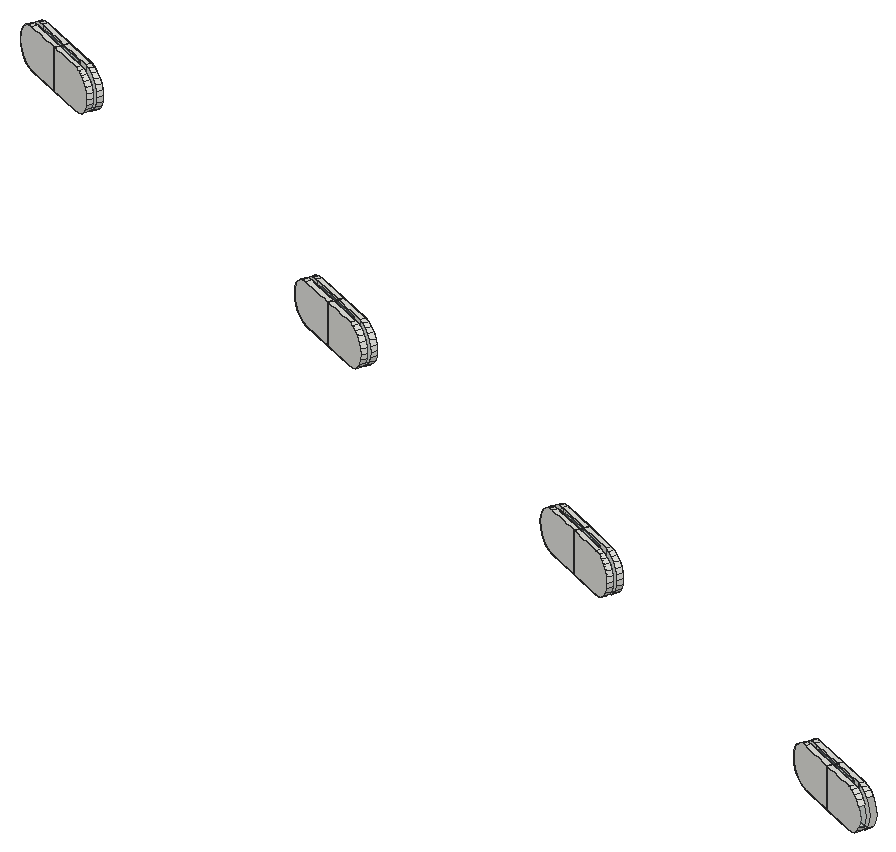
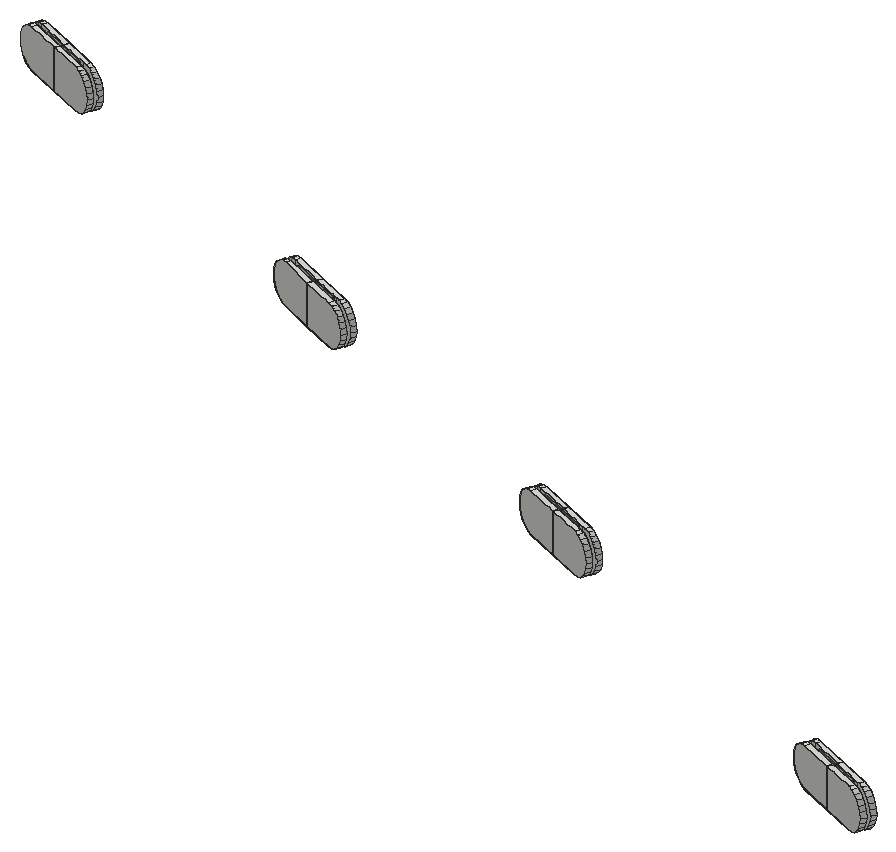
# SketchUp Ruby script. Lengths in inches.
U = 1.inch
M = Sketchup.active_model
def pt(a) = Geom::Point3d.new(a.map { |v| v * U })
def face(e, loops, mat)
  f = e.add_face(loops[0].map { |a| pt(a) })
  loops[1..].each { |l| e.add_face(l.map { |a| pt(a) }).erase! }
  f.material = f.back_material = mat if mat
  f
end
# faces: each face lists its corners as indices into pts; further lists are holes
def faces(e, pts, list, mat = nil) = list.each { |f| face(e, (f[0].is_a?(Array) ? f : [f]).map { |l| l.map { |i| pts[i] } }, mat) }
# xy, xz, yz: faces in a plane at the given z, y or x. An outline is a flat list of corners, or four numbers for a rectangle; further outlines are holes
def ring(l) = l.size == 4 ? [[l[0], l[1]], [l[2], l[1]], [l[2], l[3]], [l[0], l[3]]] : l.each_slice(2).to_a
def flat(e, list, mat, &to3) = list.each { |f| face(e, (f[0].is_a?(Array) ? f : [f]).map { |l| ring(l).map { |u, v| to3.(u, v) } }, mat) }
def xy(e, z, list, mat = nil) = flat(e, list, mat) { |x, y| [x, y, z] }
def xz(e, y, list, mat = nil) = flat(e, list, mat) { |x, z| [x, y, z] }
def yz(e, x, list, mat = nil) = flat(e, list, mat) { |y, z| [x, y, z] }
def lines(e, pts, list) = list.each { |a, b| e.add_line(pt(pts[a]), pt(pts[b])) }
# prism: a flat outline (further loops are holes) pulled along v
def prism(e, loops, v, mat = nil)
  f = face(e, loops, mat); d = Geom::Vector3d.new(v.map { |x| x * U })
  f.pushpull(f.normal.samedirection?(d) ? d.length : -d.length)
end
def box(e, o, s, mat = nil) = prism(e, [[o, [o[0] + s[0], o[1], o[2]], [o[0] + s[0], o[1] + s[1], o[2]], [o[0], o[1] + s[1], o[2]]]], [0, 0, s[2]], mat)
def at(x, y, z, deg = 0) = Geom::Transformation.translation(pt([x, y, z])) * Geom::Transformation.rotation(ORIGIN, Z_AXIS, deg.degrees)
def axes(o, x, y, z) = Geom::Transformation.new([*x, 0, *y, 0, *z, 0, *pt(o).to_a, 1])
def part(name) = M.definitions.add(name)
# library, detail: a bought-in or finely detailed component or shape, given as its bounding box
def library(name, o, s) = part(name).tap { |d| box(d.entities, o, s) }
def detail(e, o, s) = box(e.add_group.entities, o, s)
def put(e, d, t, mat = nil) = e.add_instance(d, t).tap { |i| i.material = mat if mat }
def group(e, t, mat = nil) = e.add_group.tap { |g| g.transformation = t; g.material = mat if mat }.entities
root = M.entities
M.materials.add("Glass_Safety_01").color = [204, 235, 244]
M.materials["Glass_Safety_01"].alpha = 0.1
xy(root,333,[[788.71,557.36,786.9,558.15,787.01,558.4,788.82,557.62],[788.9,557.8,787.09,558.58,787.2,558.84,789.01,558.05],[786.9,558.15,785.1,558.9375,785.21,559.1875,785.36,559.12,787.01,558.4],[787.09,558.58,785.44,559.3,785.29,559.37,785.4,559.62,787.2,558.84],[767.73,566.5,765.93,567.29,766.04,567.54,767.84,566.75],
  [767.92,566.93,766.12,567.72,766.23,567.97,768.03,567.19],[765.93,567.29,764.12,568.07,764.23,568.32,764.39,568.25,766.04,567.54],[766.12,567.72,764.47,568.43,764.3125,568.5,764.42,568.76,766.23,567.97],[747.39,575.36,745.58,576.15,745.69,576.4,747.5,575.61],[747.57,575.79,745.77,576.58,745.88,576.83,747.68,576.05],
  [745.58,576.15,743.78,576.93,743.89,577.19,744.03,577.12,745.69,576.4],[745.77,576.58,744.11,577.3,743.96,577.37,744.07,577.62,745.88,576.83],[724.68,585.25,722.875,586.04,722.99,586.29,724.79,585.5],[724.87,585.68,723.0625,586.47,723.17,586.72,724.98,585.94],[722.875,586.04,721.07,586.82,721.18,587.07,721.33,587.01,722.99,586.29],
  [723.0625,586.47,721.4,587.19,721.26,587.25,721.37,587.51,723.17,586.72]])
xy(root,333.08,[[788.46,557.77,787.01,558.4,787.09,558.58,788.54,557.95],[787.01,558.4,785.57,559.03,785.65,559.21,787.09,558.58],[767.48,566.91,766.04,567.54,766.12,567.72,767.56,567.09],[766.04,567.54,764.59,568.17,764.67,568.35,766.12,567.72],[747.13,575.77,745.69,576.4,745.77,576.58,747.21,575.95],
  [745.69,576.4,744.25,577.03,744.33,577.21,745.77,576.58],[724.43,585.66,722.99,586.29,723.0625,586.47,724.51,585.84],[722.99,586.29,721.54,586.92,721.62,587.1,723.0625,586.47]],"Glass_Safety_01")
xy(root,335.05,[[788.46,557.77,788.54,557.95,787.09,558.58,787.01,558.4],[787.01,558.4,787.09,558.58,785.65,559.21,785.57,559.03],[767.48,566.91,767.56,567.09,766.12,567.72,766.04,567.54],[766.04,567.54,766.12,567.72,764.67,568.35,764.59,568.17],[747.13,575.77,747.21,575.95,745.77,576.58,745.69,576.4],
  [745.69,576.4,745.77,576.58,744.33,577.21,744.25,577.03],[724.43,585.66,724.51,585.84,723.0625,586.47,722.99,586.29],[722.99,586.29,723.0625,586.47,721.62,587.1,721.54,586.92]],"Glass_Safety_01")
xy(root,335.125,[[788.71,557.36,788.82,557.62,787.01,558.4,786.9,558.15],[788.9,557.8,789.01,558.05,787.2,558.84,787.09,558.58],[786.9,558.15,787.01,558.4,785.36,559.12,785.21,559.1875,785.1,558.9375],[787.09,558.58,787.2,558.84,785.4,559.62,785.29,559.37,785.44,559.3],[767.73,566.5,767.84,566.75,766.04,567.54,765.93,567.29],
  [767.92,566.93,768.03,567.19,766.23,567.97,766.12,567.72],[765.93,567.29,766.04,567.54,764.39,568.25,764.23,568.32,764.12,568.07],[766.12,567.72,766.23,567.97,764.42,568.76,764.3125,568.5,764.47,568.43],[747.39,575.36,747.5,575.61,745.69,576.4,745.58,576.15],[747.57,575.79,747.68,576.05,745.88,576.83,745.77,576.58],
  [745.58,576.15,745.69,576.4,744.03,577.12,743.89,577.19,743.78,576.93],[745.77,576.58,745.88,576.83,744.07,577.62,743.96,577.37,744.11,577.3],[724.68,585.25,724.79,585.5,722.99,586.29,722.875,586.04],[724.87,585.68,724.98,585.94,723.17,586.72,723.0625,586.47],[722.875,586.04,722.99,586.29,721.33,587.01,721.18,587.07,721.07,586.82],
  [723.0625,586.47,723.17,586.72,721.37,587.51,721.26,587.25,721.4,587.19]])
p = [[788.71,557.36,335.125],[786.9,558.15,335.125],[786.9,558.15,333],[788.71,557.36,333],[788.96,557.25,333.04],[789.2,557.15,333.14],
  [789.4,557.0625,333.3125],[789.55,557,333.53],[789.65,556.95,333.79],[789.68,556.9375,334.0625],[789.65,556.95,334.34],[789.55,557,334.59],
  [789.4,557.0625,334.8125],[789.2,557.15,334.98],[788.96,557.25,335.09],[788.82,557.62,335.125],[788.82,557.62,333],[789.07,557.51,333.04],
  [789.31,557.4,333.14],[789.51,557.32,333.3125],[789.66,557.25,333.53],[789.76,557.21,333.79],[789.79,557.19,334.0625],[789.76,557.21,334.34],
  [789.66,557.25,334.59],[789.51,557.32,334.8125],[789.31,557.4,334.98],[789.07,557.51,335.09],[788.9,557.8,333],[788.9,557.8,335.125],
  [789.15,557.6875,335.09],[789.38,557.58,334.98],[789.59,557.5,334.8125],[789.74,557.43,334.59],[789.84,557.39,334.34],[789.87,557.37,334.0625],
  [789.84,557.39,333.79],[789.74,557.43,333.53],[789.59,557.5,333.3125],[789.38,557.58,333.14],[789.15,557.6875,333.04],[787.01,558.4,335.125],
  [787.01,558.4,333],[787.01,558.4,333.08],[788.46,557.77,333.08],[788.46,557.77,335.05],[787.01,558.4,335.05],[787.2,558.84,335.125],
  [789.01,558.05,335.125],[789.26,557.94,335.09],[789.49,557.84,334.98],[789.7,557.75,334.8125],[789.85,557.68,334.59],[789.95,557.64,334.34],
  [789.98,557.625,334.0625],[789.95,557.64,333.79],[789.85,557.68,333.53],[789.7,557.75,333.3125],[789.49,557.84,333.14],[789.26,557.94,333.04],
  [789.01,558.05,333],[787.2,558.84,333],[787.09,558.58,333],[787.09,558.58,335.125],[787.09,558.58,335.05],[788.54,557.95,335.05],
  [788.54,557.95,333.08],[787.09,558.58,333.08],[785.1,558.9375,335.125],[784.85,559.05,335.09],[784.61,559.15,334.98],[784.41,559.24,334.8125],
  [784.25,559.3,334.59],[784.16,559.35,334.34],[784.125,559.36,334.0625],[784.16,559.35,333.79],[784.25,559.3,333.53],[784.41,559.24,333.3125],
  [784.61,559.15,333.14],[784.85,559.05,333.04],[785.1,558.9375,333],[785.36,559.12,333],[785.36,559.12,335.125],[785.57,559.03,335.05],
  [785.57,559.03,333.08],[785.44,559.3,335.125],[785.44,559.3,333],[785.65,559.21,333.08],[785.65,559.21,335.05],[785.4,559.62,335.125],
  [785.4,559.62,333],[785.14,559.73,333.04],[784.91,559.83,333.14],[784.71,559.92,333.3125],[784.55,559.99,333.53],[784.46,560.03,333.79],
  [784.42,560.05,334.0625],[784.46,560.03,334.34],[784.55,559.99,334.59],[784.71,559.92,334.8125],[784.91,559.83,334.98],[785.14,559.73,335.09],
  [784.96,559.3,333.04],[785.21,559.1875,333],[784.72,559.4,333.14],[785.21,559.1875,335.125],[784.52,559.49,333.3125],[784.36,559.56,333.53],
  [784.27,559.6,333.79],[784.23,559.61,334.0625],[784.27,559.6,334.34],[784.36,559.56,334.59],[784.52,559.49,334.8125],[784.72,559.4,334.98],
  [784.96,559.3,335.09],[785.29,559.37,333],[785.29,559.37,335.125],[785.03,559.48,335.09],[784.8,559.58,334.98],[784.6,559.67,334.8125],
  [784.44,559.74,334.59],[784.35,559.78,334.34],[784.3125,559.79,334.0625],[784.35,559.78,333.79],[784.44,559.74,333.53],[784.6,559.67,333.3125],
  [784.8,559.58,333.14],[785.03,559.48,333.04],[767.73,566.5,335.125],[765.93,567.29,335.125],[765.93,567.29,333],[767.73,566.5,333],
  [767.98,566.39,333.04],[768.22,566.29,333.14],[768.42,566.2,333.3125],[768.58,566.13,333.53],[768.67,566.09,333.79],[768.71,566.07,334.0625],
  [768.67,566.09,334.34],[768.58,566.13,334.59],[768.42,566.2,334.8125],[768.22,566.29,334.98],[767.98,566.39,335.09],[767.84,566.75,335.125],
  [767.84,566.75,333],[768.09,566.64,333.04],[768.33,566.54,333.14],[768.53,566.45,333.3125],[768.6875,566.38,333.53],[768.78,566.34,333.79],
  [768.82,566.33,334.0625],[768.78,566.34,334.34],[768.6875,566.38,334.59],[768.53,566.45,334.8125],[768.33,566.54,334.98],[768.09,566.64,335.09],
  [767.92,566.93,333],[767.92,566.93,335.125],[768.17,566.82,335.09],[768.41,566.72,334.98],[768.61,566.63,334.8125],[768.76,566.56,334.59],
  [768.86,566.52,334.34],[768.89,566.51,334.0625],[768.86,566.52,333.79],[768.76,566.56,333.53],[768.61,566.63,333.3125],[768.41,566.72,333.14],
  [768.17,566.82,333.04],[768.28,567.08,333.04],[768.52,566.97,333.14],[766.04,567.54,335.125],[766.04,567.54,333],[766.04,567.54,333.08],
  [767.48,566.91,333.08],[767.48,566.91,335.05],[766.04,567.54,335.05],[766.23,567.97,335.125],[768.03,567.19,335.125],[768.28,567.08,335.09],
  [768.52,566.97,334.98],[768.72,566.88,334.8125],[768.875,566.82,334.59],[768.97,566.78,334.34],[769,566.76,334.0625],[768.97,566.78,333.79],
  [768.875,566.82,333.53],[768.72,566.88,333.3125],[768.03,567.19,333],[766.23,567.97,333],[766.12,567.72,333],[766.12,567.72,335.125],
  [766.12,567.72,335.05],[767.56,567.09,335.05],[767.56,567.09,333.08],[766.12,567.72,333.08],[764.12,568.07,335.125],[763.87,568.18,335.09],
  [763.63,568.28,334.98],[763.43,568.37,334.8125],[763.28,568.4375,334.59],[763.18,568.48,334.34],[763.15,568.5,334.0625],[763.18,568.48,333.79],
  [763.28,568.4375,333.53],[763.43,568.37,333.3125],[763.63,568.28,333.14],[763.87,568.18,333.04],[764.12,568.07,333],[764.39,568.25,333],
  [764.39,568.25,335.125],[764.59,568.17,335.05],[764.59,568.17,333.08],[764.47,568.43,335.125],[764.47,568.43,333],[764.67,568.35,333.08],
  [764.67,568.35,335.05],[764.42,568.76,335.125],[764.42,568.76,333],[764.17,568.87,333.04],[763.93,568.97,333.14],[763.73,569.06,333.3125],
  [763.58,569.125,333.53],[763.48,569.17,333.79],[763.45,569.18,334.0625],[763.48,569.17,334.34],[763.58,569.125,334.59],[763.73,569.06,334.8125],
  [763.93,568.97,334.98],[764.17,568.87,335.09],[763.98,568.43,333.04],[764.23,568.32,333],[763.74,568.54,333.14],[764.23,568.32,335.125],
  [763.54,568.625,333.3125],[763.39,568.69,333.53],[763.29,568.73,333.79],[763.26,568.75,334.0625],[763.29,568.73,334.34],[763.39,568.69,334.59],
  [763.54,568.625,334.8125],[763.74,568.54,334.98],[763.98,568.43,335.09],[764.3125,568.5,333],[764.3125,568.5,335.125],[764.06,568.61,335.09],
  [763.82,568.72,334.98],[763.62,568.8,334.8125],[763.47,568.87,334.59],[763.37,568.91,334.34],[763.34,568.93,334.0625],[763.37,568.91,333.79],
  [763.47,568.87,333.53],[763.62,568.8,333.3125],[763.82,568.72,333.14],[764.06,568.61,333.04],[747.39,575.36,335.125],[745.58,576.15,335.125],
  [745.58,576.15,333],[747.39,575.36,333],[747.64,575.25,333.04],[747.87,575.15,333.14],[748.07,575.0625,333.3125],[748.23,574.99,333.53],
  [748.33,574.95,333.79],[748.36,574.9375,334.0625],[748.33,574.95,334.34],[748.23,574.99,334.59],[748.07,575.0625,334.8125],[747.87,575.15,334.98],
  [747.64,575.25,335.09],[747.75,575.5,333.04],[747.98,575.4,333.14],[747.5,575.61,335.125],[747.5,575.61,333],[748.18,575.3125,333.3125],
  [748.34,575.25,333.53],[748.4375,575.2,333.79],[748.47,575.1875,334.0625],[748.4375,575.2,334.34],[748.34,575.25,334.59],[748.18,575.3125,334.8125],
  [747.98,575.4,334.98],[747.75,575.5,335.09],[747.57,575.79,333],[747.57,575.79,335.125],[747.83,575.68,335.09],[748.0625,575.58,334.98],
  [748.26,575.49,334.8125],[748.42,575.43,334.59],[748.52,575.38,334.34],[748.55,575.37,334.0625],[748.52,575.38,333.79],[748.42,575.43,333.53],
  [748.26,575.49,333.3125],[748.0625,575.58,333.14],[747.83,575.68,333.04],[745.69,576.4,335.125],[745.69,576.4,333],[745.69,576.4,333.08],
  [747.13,575.77,333.08],[747.13,575.77,335.05],[745.69,576.4,335.05],[745.88,576.83,335.125],[747.68,576.05,335.125],[747.9375,575.9375,335.09],
  [748.17,575.83,334.98],[748.375,575.75,334.8125],[748.53,575.68,334.59],[748.625,575.64,334.34],[748.66,575.62,334.0625],[748.625,575.64,333.79],
  [748.53,575.68,333.53],[748.375,575.75,333.3125],[748.17,575.83,333.14],[747.9375,575.9375,333.04],[747.68,576.05,333],[745.88,576.83,333],
  [745.77,576.58,333],[745.77,576.58,335.125],[745.77,576.58,335.05],[747.21,575.95,335.05],[747.21,575.95,333.08],[745.77,576.58,333.08],
  [743.78,576.93,335.125],[743.52,577.04,335.09],[743.29,577.15,334.98],[743.09,577.23,334.8125],[742.93,577.3,334.59],[742.83,577.34,334.34],
  [742.8,577.36,334.0625],[742.83,577.34,333.79],[742.93,577.3,333.53],[743.09,577.23,333.3125],[743.29,577.15,333.14],[743.52,577.04,333.04],
  [743.78,576.93,333],[744.03,577.12,333],[744.03,577.12,335.125],[744.25,577.03,335.05],[744.25,577.03,333.08],[744.11,577.3,335.125],
  [744.11,577.3,333],[744.33,577.21,333.08],[744.33,577.21,335.05],[744.07,577.62,335.125],[744.07,577.62,333],[743.82,577.73,333.04],
  [743.59,577.83,333.14],[743.39,577.92,333.3125],[743.23,577.99,333.53],[743.13,578.03,333.79],[743.1,578.04,334.0625],[743.13,578.03,334.34],
  [743.23,577.99,334.59],[743.39,577.92,334.8125],[743.59,577.83,334.98],[743.82,577.73,335.09],[743.63,577.3,333.04],[743.89,577.19,333],
  [743.4,577.4,333.14],[743.89,577.19,335.125],[743.2,577.49,333.3125],[743.04,577.55,333.53],[742.94,577.6,333.79],[742.91,577.61,334.0625],
  [742.94,577.6,334.34],[743.04,577.55,334.59],[743.2,577.49,334.8125],[743.4,577.4,334.98],[743.63,577.3,335.09],[743.96,577.37,333],
  [743.96,577.37,335.125],[743.71,577.48,335.09],[743.48,577.58,334.98],[743.28,577.67,334.8125],[743.12,577.73,334.59],[743.02,577.78,334.34],
  [742.99,577.79,334.0625],[743.02,577.78,333.79],[743.12,577.73,333.53],[743.28,577.67,333.3125],[743.48,577.58,333.14],[743.71,577.48,333.04],
  [724.68,585.25,335.125],[722.875,586.04,335.125],[722.875,586.04,333],[724.68,585.25,333],[724.93,585.14,333.04],[725.17,585.04,333.14],
  [725.37,584.95,333.3125],[725.52,584.88,333.53],[725.62,584.84,333.79],[725.65,584.83,334.0625],[725.62,584.84,334.34],[725.52,584.88,334.59],
  [725.37,584.95,334.8125],[725.17,585.04,334.98],[724.93,585.14,335.09],[725.04,585.39,333.04],[725.28,585.29,333.14],[724.79,585.5,333],
  [724.79,585.5,335.125],[725.48,585.2,333.3125],[725.63,585.13,333.53],[725.73,585.09,333.79],[725.76,585.08,334.0625],[725.73,585.09,334.34],
  [725.63,585.13,334.59],[725.48,585.2,334.8125],[725.28,585.29,334.98],[725.04,585.39,335.09],[724.87,585.68,333],[724.87,585.68,335.125],
  [725.12,585.57,335.09],[725.36,585.47,334.98],[725.56,585.38,334.8125],[725.71,585.32,334.59],[725.81,585.27,334.34],[725.84,585.26,334.0625],
  [725.81,585.27,333.79],[725.71,585.32,333.53],[725.56,585.38,333.3125],[725.36,585.47,333.14],[725.12,585.57,333.04],[722.99,586.29,335.125],
  [722.99,586.29,333],[722.99,586.29,333.08],[724.43,585.66,333.08],[724.43,585.66,335.05],[722.99,586.29,335.05],[723.17,586.72,335.125],
  [724.98,585.94,335.125],[725.23,585.83,335.09],[725.47,585.72,334.98],[725.67,585.64,334.8125],[725.82,585.57,334.59],[725.92,585.53,334.34],
  [725.95,585.51,334.0625],[725.92,585.53,333.79],[725.82,585.57,333.53],[725.67,585.64,333.3125],[725.47,585.72,333.14],[725.23,585.83,333.04],
  [724.98,585.94,333],[723.17,586.72,333],[723.0625,586.47,333],[723.0625,586.47,335.125],[723.0625,586.47,335.05],[724.51,585.84,335.05],
  [724.51,585.84,333.08],[723.0625,586.47,333.08],[721.07,586.82,335.125],[720.82,586.93,335.09],[720.58,587.03,334.98],[720.38,587.12,334.8125],
  [720.23,587.1875,334.59],[720.13,587.23,334.34],[720.1,587.25,334.0625],[720.13,587.23,333.79],[720.23,587.1875,333.53],[720.38,587.12,333.3125],
  [720.58,587.03,333.14],[720.82,586.93,333.04],[721.07,586.82,333],[721.33,587.01,333],[721.33,587.01,335.125],[721.54,586.92,335.05],
  [721.54,586.92,333.08],[721.4,587.19,335.125],[721.4,587.19,333],[721.62,587.1,333.08],[721.62,587.1,335.05],[721.37,587.51,335.125],
  [721.37,587.51,333],[721.12,587.62,333.04],[720.88,587.72,333.14],[720.68,587.81,333.3125],[720.53,587.875,333.53],[720.43,587.92,333.79],
  [720.39,587.93,334.0625],[720.43,587.92,334.34],[720.53,587.875,334.59],[720.68,587.81,334.8125],[720.88,587.72,334.98],[721.12,587.62,335.09],
  [720.93,587.18,333.04],[721.18,587.07,333],[720.69,587.29,333.14],[721.18,587.07,335.125],[720.49,587.375,333.3125],[720.34,587.44,333.53],
  [720.24,587.48,333.79],[720.21,587.5,334.0625],[720.24,587.48,334.34],[720.34,587.44,334.59],[720.49,587.375,334.8125],[720.69,587.29,334.98],
  [720.93,587.18,335.09],[721.26,587.25,333],[721.26,587.25,335.125],[721.01,587.36,335.09],[720.77,587.47,334.98],[720.57,587.55,334.8125],
  [720.42,587.62,334.59],[720.32,587.66,334.34],[720.28,587.68,334.0625],[720.32,587.66,333.79],[720.42,587.62,333.53],[720.57,587.55,333.3125],
  [720.77,587.47,333.14],[721.01,587.36,333.04]]
faces(root,p,[[0,1,2,3,4,5,6,7,8,9,10,11,12,13,14],[17,18,5,4],[16,17,4,3],[41,15,16,42,43,44,45,46],[47,48,49,50,51,52,53,54,55,56,57,58,59,60,61],[39,40,59,58],[40,28,60,59],[62,28,29,63,64,65,66,67],
  [1,68,69,70,71,72,73,74,75,76,77,78,79,80,2],[42,43,46,41,1,2],[42,81,82,41,46,83,84,43],[63,85,86,62,67,87,88,64],[67,62,61,47,63,64],[89,47,61,90,91,92,93,94,95,96,97,98,99,100,101],[102,103,80,79],[104,102,79,78],
  [105,82,81,103,102,104,106,107,108,109,110,111,112,113,114],[115,86,85,116,117,118,119,120,121,122,123,124,125,126,127],[115,127,91,90],[127,126,92,91],[128,129,130,131,132,133,134,135,136,137,138,139,140,141,142],[145,146,133,132],[144,145,132,131],[167,168,169,170],
  [171,143,144,172,173,174,175,176],[177,178,179,180,181,182,183,184,185,186,187,170,169,188,189],[168,156,188,169],[190,156,157,191,192,193,194,195],[129,196,197,198,199,200,201,202,203,204,205,206,207,208,130],[172,173,176,171,129,130],[172,209,210,171,176,211,212,173],[191,213,214,190,195,215,216,192],
  [195,190,189,177,191,192],[217,177,189,218,219,220,221,222,223,224,225,226,227,228,229],[230,231,208,207],[232,230,207,206],[233,210,209,231,230,232,234,235,236,237,238,239,240,241,242],[243,214,213,244,245,246,247,248,249,250,251,252,253,254,255],[243,255,219,218],[255,254,220,219],
  [256,257,258,259,260,261,262,263,264,265,266,267,268,269,270],[271,272,261,260],[274,271,260,259],[297,273,274,298,299,300,301,302],[303,304,305,306,307,308,309,310,311,312,313,314,315,316,317],[295,296,315,314],[296,284,316,315],[318,284,285,319,320,321,322,323],
  [257,324,325,326,327,328,329,330,331,332,333,334,335,336,258],[298,299,302,297,257,258],[298,337,338,297,302,339,340,299],[319,341,342,318,323,343,344,320],[323,318,317,303,319,320],[345,303,317,346,347,348,349,350,351,352,353,354,355,356,357],[358,359,336,335],[360,358,335,334],
  [361,338,337,359,358,360,362,363,364,365,366,367,368,369,370],[371,342,341,372,373,374,375,376,377,378,379,380,381,382,383],[371,383,347,346],[383,382,348,347],[384,385,386,387,388,389,390,391,392,393,394,395,396,397,398],[399,400,389,388],[401,399,388,387],[425,402,401,426,427,428,429,430],
  [431,432,433,434,435,436,437,438,439,440,441,442,443,444,445],[423,424,443,442],[424,412,444,443],[446,412,413,447,448,449,450,451],[385,452,453,454,455,456,457,458,459,460,461,462,463,464,386],[426,427,430,425,385,386],[426,465,466,425,430,467,468,427],[447,469,470,446,451,471,472,448],
  [451,446,445,431,447,448],[473,431,445,474,475,476,477,478,479,480,481,482,483,484,485],[486,487,464,463],[488,486,463,462],[489,466,465,487,486,488,490,491,492,493,494,495,496,497,498],[499,470,469,500,501,502,503,504,505,506,507,508,509,510,511],[499,511,475,474],[511,510,476,475],
  [18,19,6,5],[38,39,58,57],[106,104,78,77],[126,125,93,92],[146,147,134,133],[166,167,170,187],[234,232,206,205],[254,253,221,220],
  [272,275,262,261],[294,295,314,313],[362,360,334,333],[382,381,349,348],[400,403,390,389],[422,423,442,441],[490,488,462,461],[510,509,477,476],
  [19,20,7,6],[107,106,77,76],[125,124,94,93],[147,148,135,134],[165,166,187,186],[235,234,205,204],[253,252,222,221],[275,276,263,262],
  [293,294,313,312],[363,362,333,332],[381,380,350,349],[403,404,391,390],[421,422,441,440],[491,490,461,460],[509,508,478,477],[108,107,76,75],
  [124,123,95,94],[148,149,136,135],[164,165,186,185],[236,235,204,203],[252,251,223,222],[276,277,264,263],[292,293,312,311],[364,363,332,331],
  [380,379,351,350],[404,405,392,391],[420,421,440,439],[492,491,460,459],[508,507,479,478],[109,108,75,74],[123,122,96,95],[149,150,137,136],
  [163,164,185,184],[237,236,203,202],[251,250,224,223],[277,278,265,264],[291,292,311,310],[365,364,331,330],[379,378,352,351],[405,406,393,392],
  [419,420,439,438],[507,506,480,479],[110,109,74,73],[122,121,97,96],[150,151,138,137],[162,163,184,183],[238,237,202,201],[250,249,225,224],
  [278,279,266,265],[290,291,310,309],[366,365,330,329],[378,377,353,352],[406,407,394,393],[418,419,438,437],[494,493,458,457],[506,505,481,480],
  [111,110,73,72],[121,120,98,97],[151,152,139,138],[161,162,183,182],[239,238,201,200],[249,248,226,225],[279,280,267,266],[289,290,309,308],
  [367,366,329,328],[377,376,354,353],[407,408,395,394],[417,418,437,436],[495,494,457,456],[505,504,482,481],[24,25,12,11],[112,111,72,71],
  [120,119,99,98],[152,153,140,139],[160,161,182,181],[240,239,200,199],[248,247,227,226],[280,281,268,267],[288,289,308,307],[368,367,328,327],
  [376,375,355,354],[408,409,396,395],[416,417,436,435],[496,495,456,455],[504,503,483,482],[25,26,13,12],[31,32,51,50],[113,112,71,70],
  [119,118,100,99],[153,154,141,140],[159,160,181,180],[241,240,199,198],[247,246,228,227],[281,282,269,268],[287,288,307,306],[369,368,327,326],
  [375,374,356,355],[409,410,397,396],[415,416,435,434],[497,496,455,454],[503,502,484,483],[26,27,14,13],[30,31,50,49],[114,113,70,69],
  [118,117,101,100],[154,155,142,141],[158,159,180,179],[242,241,198,197],[246,245,229,228],[282,283,270,269],[286,287,306,305],[370,369,326,325],
  [374,373,357,356],[410,411,398,397],[414,415,434,433],[498,497,454,453],[502,501,485,484],[27,15,0,14],[29,30,49,48],[105,114,69,68],
  [117,116,89,101],[155,143,128,142],[157,158,179,178],[233,242,197,196],[245,244,217,229],[283,273,256,270],[285,286,305,304],[361,370,325,324],
  [373,372,345,357],[411,402,384,398],[413,414,433,432],[489,498,453,452],[501,500,473,485]])
faces(root,p,[[15,16,17,18,19,20,21,22,23,24,25,26,27],[28,29,30,31,32,33,34,35,36,37,38,39,40],[143,144,145,146,147,148,149,150,151,152,153,154,155],[156,157,158,159,160,161,162,163,164,165,166,167,168],[273,274,271,272,275,276,277,278,279,280,281,282,283],[284,285,286,287,288,289,290,291,292,293,294,295,296],[402,401,399,400,403,404,405,406,407,408,409,410,411],[412,413,414,415,416,417,418,419,420,421,422,423,424],
  [44,43,46,45],[45,44,66,65],[67,66,65,64],[43,84,83,46],[64,46,43,67],[87,67,64,88],[84,83,88,87],[174,173,176,175],
  [175,174,194,193],[195,194,193,192],[173,212,211,176],[192,176,173,195],[215,195,192,216],[212,211,216,215],[300,299,302,301],[301,300,322,321],
  [323,322,321,320],[299,340,339,302],[320,302,299,323],[343,323,320,344],[340,339,344,343],[428,427,430,429],[450,449,429,428],[451,450,449,448],
  [427,468,467,430],[427,451,448,430],[471,451,448,472],[468,467,472,471]],"Glass_Safety_01")
